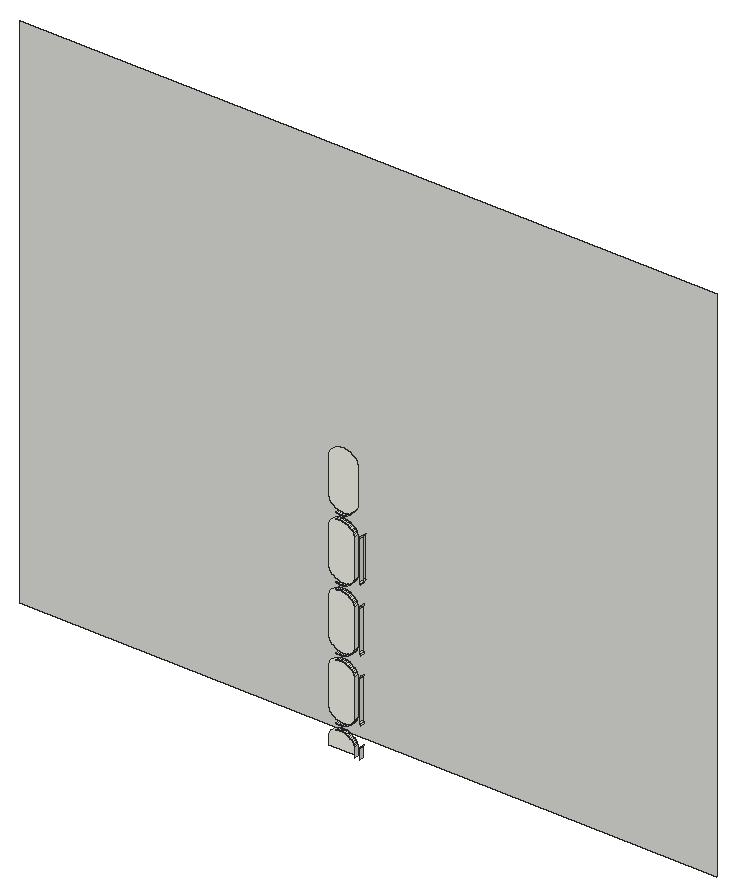
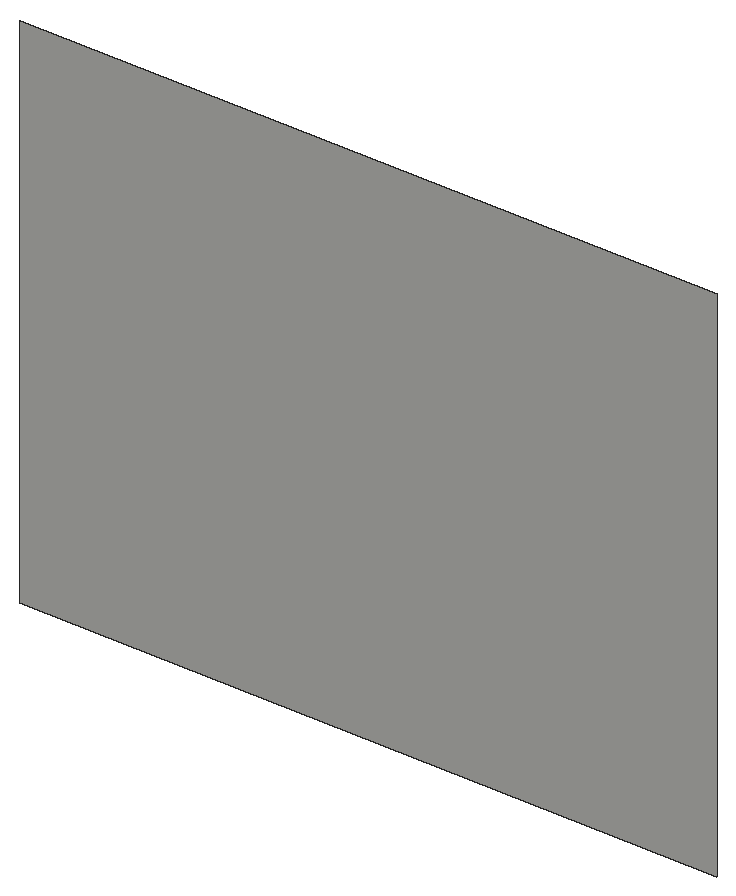
# SketchUp Ruby script. Lengths in inches.
U = 1.inch
M = Sketchup.active_model
def pt(a) = Geom::Point3d.new(a.map { |v| v * U })
def face(e, loops, mat)
  f = e.add_face(loops[0].map { |a| pt(a) })
  loops[1..].each { |l| e.add_face(l.map { |a| pt(a) }).erase! }
  f.material = f.back_material = mat if mat
  f
end
# faces: each face lists its corners as indices into pts; further lists are holes
def faces(e, pts, list, mat = nil) = list.each { |f| face(e, (f[0].is_a?(Array) ? f : [f]).map { |l| l.map { |i| pts[i] } }, mat) }
# xy, xz, yz: faces in a plane at the given z, y or x. An outline is a flat list of corners, or four numbers for a rectangle; further outlines are holes
def ring(l) = l.size == 4 ? [[l[0], l[1]], [l[2], l[1]], [l[2], l[3]], [l[0], l[3]]] : l.each_slice(2).to_a
def flat(e, list, mat, &to3) = list.each { |f| face(e, (f[0].is_a?(Array) ? f : [f]).map { |l| ring(l).map { |u, v| to3.(u, v) } }, mat) }
def xy(e, z, list, mat = nil) = flat(e, list, mat) { |x, y| [x, y, z] }
def xz(e, y, list, mat = nil) = flat(e, list, mat) { |x, z| [x, y, z] }
def yz(e, x, list, mat = nil) = flat(e, list, mat) { |y, z| [x, y, z] }
def lines(e, pts, list) = list.each { |a, b| e.add_line(pt(pts[a]), pt(pts[b])) }
# prism: a flat outline (further loops are holes) pulled along v
def prism(e, loops, v, mat = nil)
  f = face(e, loops, mat); d = Geom::Vector3d.new(v.map { |x| x * U })
  f.pushpull(f.normal.samedirection?(d) ? d.length : -d.length)
end
def box(e, o, s, mat = nil) = prism(e, [[o, [o[0] + s[0], o[1], o[2]], [o[0] + s[0], o[1] + s[1], o[2]], [o[0], o[1] + s[1], o[2]]]], [0, 0, s[2]], mat)
def at(x, y, z, deg = 0) = Geom::Transformation.translation(pt([x, y, z])) * Geom::Transformation.rotation(ORIGIN, Z_AXIS, deg.degrees)
def axes(o, x, y, z) = Geom::Transformation.new([*x, 0, *y, 0, *z, 0, *pt(o).to_a, 1])
def part(name) = M.definitions.add(name)
# library, detail: a bought-in or finely detailed component or shape, given as its bounding box
def library(name, o, s) = part(name).tap { |d| box(d.entities, o, s) }
def detail(e, o, s) = box(e.add_group.entities, o, s)
def put(e, d, t, mat = nil) = e.add_instance(d, t).tap { |i| i.material = mat if mat }
def group(e, t, mat = nil) = e.add_group.tap { |g| g.transformation = t; g.material = mat if mat }.entities
root = M.entities
M.materials.add("Tafisa-Gardenia-or-Gardenia-PM775-4K").color = [246, 245, 235]
xz(root,138.79,[[72.5,6,78.5,6,78.5,8,78.36,8.29,78.2,8.56,78.01,8.82,77.79,9.05,77.56,9.26,77.3,9.45,77.03,9.62,76.74,9.75,76.44,9.86,76.13,9.9375,75.82,9.98,75.5,10,75.18,9.98,74.87,9.9375,74.56,9.86,74.26,9.75,73.97,9.62,73.7,9.45,73.44,9.26,73.21,9.05,72.99,8.82,72.8,8.56,72.64,8.29,72.5,8],[75.5,11,75.82,11.02,76.13,11.0625,76.44,11.14,76.74,11.25,77.03,11.38,77.3,11.55,77.56,11.74,77.79,11.95,78.01,12.18,78.2,12.44,78.36,12.71,78.5,13,78.5,21,78.36,21.29,78.2,21.56,78.01,21.82,77.79,22.05,77.56,22.26,77.3,22.45,77.03,22.62,76.74,22.75,76.44,22.86,76.13,22.9375,75.82,22.98,75.5,23,75.18,22.98,74.87,22.9375,74.56,22.86,74.26,22.75,73.97,22.62,73.7,22.45,73.44,22.26,73.21,22.05,72.99,21.82,72.8,21.56,72.64,21.29,72.5,21,72.5,13,72.64,12.71,72.8,12.44,72.99,12.18,73.21,11.95,73.44,11.74,73.7,11.55,73.97,11.38,74.26,11.25,74.56,11.14,74.87,11.0625,75.18,11.02],[75.5,24,75.82,24.02,76.13,24.0625,76.44,24.14,76.74,24.25,77.03,24.38,77.3,24.55,77.56,24.74,77.79,24.95,78.01,25.18,78.2,25.44,78.36,25.71,78.5,26,78.5,34,78.36,34.29,78.2,34.56,78.01,34.82,77.79,35.05,77.56,35.26,77.3,35.45,77.03,35.62,76.74,35.75,76.44,35.86,76.13,35.9375,75.82,35.98,75.5,36,75.18,35.98,74.87,35.9375,74.56,35.86,74.26,35.75,73.97,35.62,73.7,35.45,73.44,35.26,73.21,35.05,72.99,34.82,72.8,34.56,72.64,34.29,72.5,34,72.5,26,72.64,25.71,72.8,25.44,72.99,25.18,73.21,24.95,73.44,24.74,73.7,24.55,73.97,24.38,74.26,24.25,74.56,24.14,74.87,24.0625,75.18,24.02],[75.5,37,75.82,37.02,76.13,37.0625,76.44,37.14,76.74,37.25,77.03,37.38,77.3,37.55,77.56,37.74,77.79,37.95,78.01,38.18,78.2,38.44,78.36,38.71,78.5,39,78.5,47,78.36,47.29,78.2,47.56,78.01,47.82,77.79,48.05,77.56,48.26,77.3,48.45,77.03,48.62,76.74,48.75,76.44,48.86,76.13,48.9375,75.82,48.98,75.5,49,75.18,48.98,74.87,48.9375,74.56,48.86,74.26,48.75,73.97,48.62,73.7,48.45,73.44,48.26,73.21,48.05,72.99,47.82,72.8,47.56,72.64,47.29,72.5,47,72.5,39,72.64,38.71,72.8,38.44,72.99,38.18,73.21,37.95,73.44,37.74,73.7,37.55,73.97,37.38,74.26,37.25,74.56,37.14,74.87,37.0625,75.18,37.02],[75.5,50,75.82,50.02,76.13,50.0625,76.44,50.14,76.74,50.25,77.03,50.38,77.3,50.55,77.56,50.74,77.79,50.95,78.01,51.18,78.2,51.44,78.36,51.71,78.5,52,78.5,60,78.36,60.29,78.2,60.56,78.01,60.82,77.79,61.05,77.56,61.26,77.3,61.45,77.03,61.62,76.74,61.75,76.44,61.86,76.13,61.9375,75.82,61.98,75.5,62,75.18,61.98,74.87,61.9375,74.56,61.86,74.26,61.75,73.97,61.62,73.7,61.45,73.44,61.26,73.21,61.05,72.99,60.82,72.8,60.56,72.64,60.29,72.5,60,72.5,52,72.64,51.71,72.8,51.44,72.99,51.18,73.21,50.95,73.44,50.74,73.7,50.55,73.97,50.38,74.26,50.25,74.56,50.14,74.87,50.0625,75.18,50.02]],"Tafisa-Gardenia-or-Gardenia-PM775-4K")
xz(root,144,[[4.5,6,148.5,114]])
yz(root,78.5,[[138,6,138.79,8],[138,13,138.79,21],[138,26,138.79,34],[138,39,138.79,47]])
yz(root,79.5,[[138,6,138.79,8],[138,13,138.79,21],[138,26,138.79,34],[138,39,138.79,47],[138.79,39,139.4375,47]])
p = [[78.36,138.79,8.29],[78.5,138.79,8],[78.5,138,8],[78.36,138,8.29],[79.5,138.79,8],[79.64,138.79,8.29],
  [79.64,138,8.29],[79.5,138,8],[78.2,138.79,8.56],[78.2,138,8.56],[79.8,138.79,8.56],[79.8,138,8.56],
  [78.01,138.79,8.82],[78.01,138,8.82],[77.79,138.79,9.05],[77.79,138,9.05],[77.56,138.79,9.26],[77.56,138,9.26],
  [77.3,138.79,9.45],[77.3,138,9.45],[77.03,138.79,9.62],[77.03,138,9.62],[76.74,138.79,9.75],[76.74,138,9.75],
  [76.44,138.79,9.86],[76.44,138,9.86],[74.56,138.79,9.86],[74.87,138.79,9.9375],[74.87,138,9.9375],[74.56,138,9.86],
  [75.18,138.79,9.98],[75.18,138,9.98],[75.82,138.79,9.98],[76.13,138.79,9.9375],[76.13,138,9.9375],[75.82,138,9.98],
  [75.5,138.79,10],[75.5,138,10],[75.18,138.79,11.02],[74.87,138.79,11.0625],[74.87,138,11.0625],[75.18,138,11.02],
  [75.5,138.79,11],[75.5,138,11],[75.82,138.79,11.02],[75.82,138,11.02],[76.13,138.79,11.0625],[76.13,138,11.0625],
  [74.56,138.79,11.14],[74.56,138,11.14],[76.44,138.79,11.14],[76.44,138,11.14],[76.74,138.79,11.25],[76.74,138,11.25],
  [77.03,138.79,11.38],[77.03,138,11.38],[77.3,138.79,11.55],[77.3,138,11.55],[77.56,138.79,11.74],[77.56,138,11.74],
  [77.79,138.79,11.95],[77.79,138,11.95],[78.01,138.79,12.18],[78.01,138,12.18],[78.2,138.79,12.44],[78.2,138,12.44],
  [78.36,138.79,12.71],[78.36,138,12.71],[79.8,138.79,12.44],[79.64,138.79,12.71],[79.64,138,12.71],[79.8,138,12.44],
  [78.5,138.79,13],[78.5,138,13],[79.5,138.79,13],[79.5,138,13],[78.36,138.79,21.29],[78.5,138.79,21],
  [78.5,138,21],[78.36,138,21.29],[79.5,138.79,21],[79.64,138.79,21.29],[79.64,138,21.29],[79.5,138,21],
  [78.2,138.79,21.56],[78.2,138,21.56],[79.8,138.79,21.56],[79.8,138,21.56],[78.01,138.79,21.82],[78.01,138,21.82],
  [77.79,138.79,22.05],[77.79,138,22.05],[77.56,138.79,22.26],[77.56,138,22.26],[77.3,138.79,22.45],[77.3,138,22.45],
  [77.03,138.79,22.62],[77.03,138,22.62],[76.74,138.79,22.75],[76.74,138,22.75],[76.44,138.79,22.86],[76.44,138,22.86],
  [74.56,138.79,22.86],[74.87,138.79,22.9375],[74.87,138,22.9375],[74.56,138,22.86],[75.18,138.79,22.98],[75.18,138,22.98],
  [75.82,138.79,22.98],[76.13,138.79,22.9375],[76.13,138,22.9375],[75.82,138,22.98],[75.5,138.79,23],[75.5,138,23],
  [75.18,138.79,24.02],[74.87,138.79,24.0625],[74.87,138,24.0625],[75.18,138,24.02],[75.5,138.79,24],[75.5,138,24],
  [75.82,138.79,24.02],[75.82,138,24.02],[76.13,138.79,24.0625],[76.13,138,24.0625],[74.56,138.79,24.14],[74.56,138,24.14],
  [76.44,138.79,24.14],[76.44,138,24.14],[76.74,138.79,24.25],[76.74,138,24.25],[77.03,138.79,24.38],[77.03,138,24.38],
  [77.3,138.79,24.55],[77.3,138,24.55],[77.56,138.79,24.74],[77.56,138,24.74],[77.79,138.79,24.95],[77.79,138,24.95],
  [78.01,138.79,25.18],[78.01,138,25.18],[78.2,138.79,25.44],[78.2,138,25.44],[78.36,138.79,25.71],[78.36,138,25.71],
  [79.8,138.79,25.44],[79.64,138.79,25.71],[79.64,138,25.71],[79.8,138,25.44],[78.5,138.79,26],[78.5,138,26],
  [79.5,138.79,26],[79.5,138,26],[78.36,138.79,34.29],[78.5,138.79,34],[78.5,138,34],[78.36,138,34.29],
  [79.5,138.79,34],[79.64,138.79,34.29],[79.64,138,34.29],[79.5,138,34],[78.2,138.79,34.56],[78.2,138,34.56],
  [79.8,138.79,34.56],[79.8,138,34.56],[78.01,138.79,34.82],[78.01,138,34.82],[77.79,138.79,35.05],[77.79,138,35.05],
  [77.56,138.79,35.26],[77.56,138,35.26],[77.3,138.79,35.45],[77.3,138,35.45],[77.03,138.79,35.62],[77.03,138,35.62],
  [76.74,138.79,35.75],[76.74,138,35.75],[76.44,138.79,35.86],[76.44,138,35.86],[74.56,138.79,35.86],[74.87,138.79,35.9375],
  [74.87,138,35.9375],[74.56,138,35.86],[75.18,138.79,35.98],[75.18,138,35.98],[75.82,138.79,35.98],[76.13,138.79,35.9375],
  [76.13,138,35.9375],[75.82,138,35.98],[75.5,138.79,36],[75.5,138,36],[75.18,138.79,37.02],[74.87,138.79,37.0625],
  [74.87,138,37.0625],[75.18,138,37.02],[75.5,138.79,37],[75.5,138,37],[75.82,138.79,37.02],[75.82,138,37.02],
  [76.13,138.79,37.0625],[76.13,138,37.0625],[74.56,138.79,37.14],[74.56,138,37.14],[76.44,138.79,37.14],[76.44,138,37.14],
  [76.74,138.79,37.25],[76.74,138,37.25],[77.03,138.79,37.38],[77.03,138,37.38],[77.3,138.79,37.55],[77.3,138,37.55],
  [77.56,138.79,37.74],[77.56,138,37.74],[77.79,138.79,37.95],[77.79,138,37.95],[78.01,138.79,38.18],[78.01,138,38.18],
  [78.2,138.79,38.44],[78.2,138,38.44],[78.36,138.79,38.71],[78.36,138,38.71],[79.8,138.79,38.44],[79.64,138.79,38.71],
  [79.64,138,38.71],[79.8,138,38.44],[78.5,138.79,39],[78.5,138,39],[79.5,138.79,39],[79.5,138,39],
  [79.5,139.4375,39],[79.64,139.4375,38.71],[78.36,138.79,47.29],[78.5,138.79,47],[78.5,138,47],[78.36,138,47.29],
  [79.5,138.79,47],[79.64,138.79,47.29],[79.64,138,47.29],[79.5,138,47],[79.64,139.4375,47.29],[79.5,139.4375,47],
  [78.2,138.79,47.56],[78.2,138,47.56],[78.01,138.79,47.82],[78.01,138,47.82],[77.79,138.79,48.05],[77.79,138,48.05],
  [77.56,138.79,48.26],[77.56,138,48.26],[77.3,138.79,48.45],[77.3,138,48.45],[77.03,138.79,48.62],[77.03,138,48.62],
  [76.74,138.79,48.75],[76.74,138,48.75],[76.44,138.79,48.86],[76.44,138,48.86],[74.56,138.79,48.86],[74.87,138.79,48.9375],
  [74.87,138,48.9375],[74.56,138,48.86],[75.18,138.79,48.98],[75.18,138,48.98],[75.82,138.79,48.98],[76.13,138.79,48.9375],
  [76.13,138,48.9375],[75.82,138,48.98],[75.5,138.79,49],[75.5,138,49],[75.18,138.79,50.02],[74.87,138.79,50.0625],
  [74.87,138,50.0625],[75.18,138,50.02],[75.5,138.79,50],[75.5,138,50],[75.82,138.79,50.02],[75.82,138,50.02],
  [76.13,138.79,50.0625],[76.13,138,50.0625],[74.56,138.79,50.14],[74.56,138,50.14],[76.44,138.79,50.14],[76.44,138,50.14],
  [76.74,138.79,50.25],[76.74,138,50.25],[77.03,138.79,50.38],[77.03,138,50.38],[77.3,138.79,50.55],[77.3,138,50.55],
  [77.56,138.79,50.74],[77.56,138,50.74],[77.79,138.79,50.95],[77.79,138,50.95],[78.01,138.79,51.18],[78.01,138,51.18],
  [78.2,138.79,51.44],[78.2,138,51.44]]
faces(root,p,[[0,1,2,3],[4,5,6,7],[8,0,3,9],[5,10,11,6],[12,8,9,13],[14,12,13,15],[16,14,15,17],[18,16,17,19],
  [20,18,19,21],[22,20,21,23],[24,22,23,25],[26,27,28,29],[27,30,31,28],[32,33,34,35],[33,24,25,34],[30,36,37,31],
  [36,32,35,37],[38,39,40,41],[42,38,41,43],[44,42,43,45],[46,44,45,47],[39,48,49,40],[50,46,47,51],[52,50,51,53],
  [54,52,53,55],[56,54,55,57],[58,56,57,59],[60,58,59,61],[62,60,61,63],[64,62,63,65],[66,64,65,67],[68,69,70,71],
  [72,66,67,73],[69,74,75,70],[76,77,78,79],[80,81,82,83],[84,76,79,85],[81,86,87,82],[88,84,85,89],[90,88,89,91],
  [92,90,91,93],[94,92,93,95],[96,94,95,97],[98,96,97,99],[100,98,99,101],[102,103,104,105],[103,106,107,104],[108,109,110,111],
  [109,100,101,110],[106,112,113,107],[112,108,111,113],[114,115,116,117],[118,114,117,119],[120,118,119,121],[122,120,121,123],[115,124,125,116],
  [126,122,123,127],[128,126,127,129],[130,128,129,131],[132,130,131,133],[134,132,133,135],[136,134,135,137],[138,136,137,139],[140,138,139,141],
  [142,140,141,143],[144,145,146,147],[148,142,143,149],[145,150,151,146],[152,153,154,155],[156,157,158,159],[160,152,155,161],[157,162,163,158],
  [164,160,161,165],[166,164,165,167],[168,166,167,169],[170,168,169,171],[172,170,171,173],[174,172,173,175],[176,174,175,177],[178,179,180,181],
  [179,182,183,180],[184,185,186,187],[185,176,177,186],[182,188,189,183],[188,184,187,189],[190,191,192,193],[194,190,193,195],[196,194,195,197],
  [198,196,197,199],[191,200,201,192],[202,198,199,203],[204,202,203,205],[206,204,205,207],[208,206,207,209],[210,208,209,211],[212,210,211,213],
  [214,212,213,215],[216,214,215,217],[218,216,217,219],[220,221,222,223],[224,218,219,225],[221,226,227,222],[228,226,221,229],[230,231,232,233],
  [234,235,236,237],[238,235,234,239],[240,230,233,241],[242,240,241,243],[244,242,243,245],[246,244,245,247],[248,246,247,249],[250,248,249,251],
  [252,250,251,253],[254,252,253,255],[256,257,258,259],[257,260,261,258],[262,263,264,265],[263,254,255,264],[260,266,267,261],[266,262,265,267],
  [268,269,270,271],[272,268,271,273],[274,272,273,275],[276,274,275,277],[269,278,279,270],[280,276,277,281],[282,280,281,283],[284,282,283,285],
  [286,284,285,287],[288,286,287,289],[290,288,289,291],[292,290,291,293],[294,292,293,295]])
